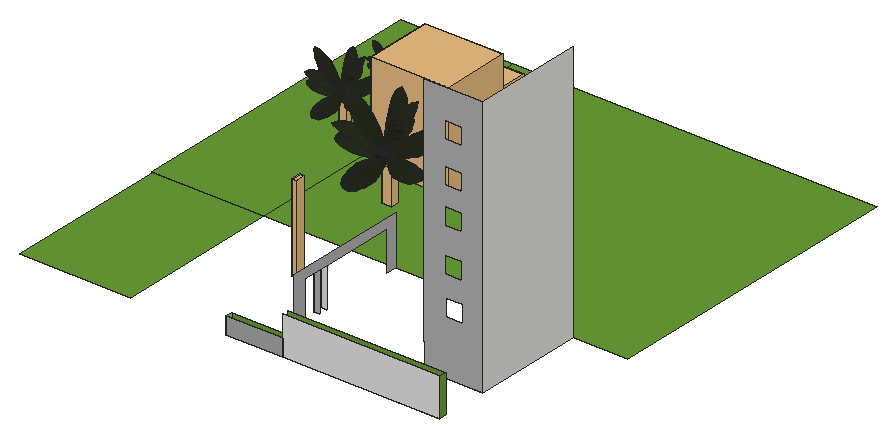
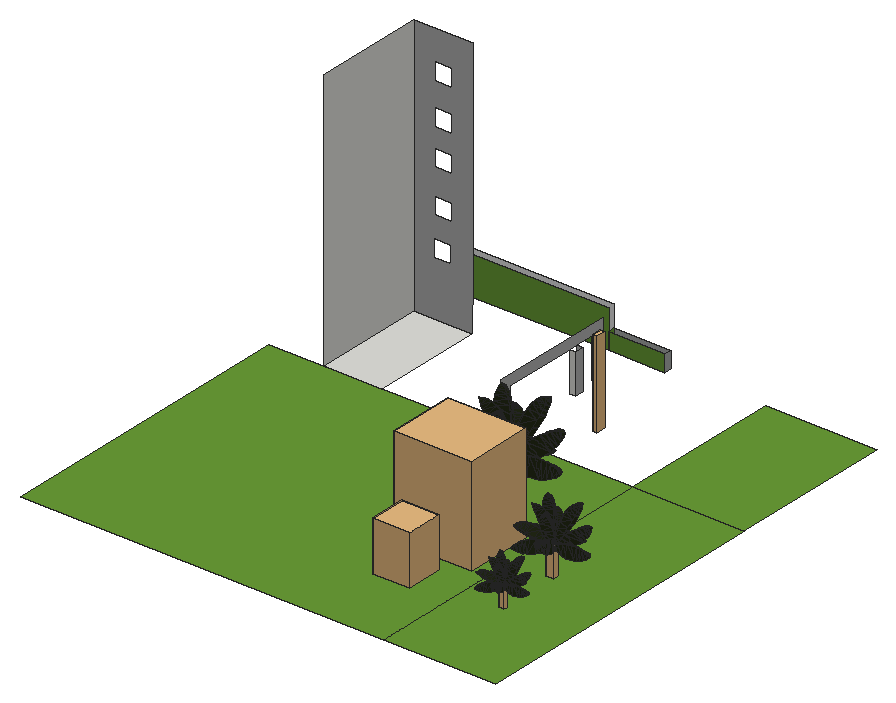
# SketchUp Ruby script. Lengths in inches.
U = 1.inch
M = Sketchup.active_model
def pt(a) = Geom::Point3d.new(a.map { |v| v * U })
def face(e, loops, mat)
  f = e.add_face(loops[0].map { |a| pt(a) })
  loops[1..].each { |l| e.add_face(l.map { |a| pt(a) }).erase! }
  f.material = f.back_material = mat if mat
  f
end
# faces: each face lists its corners as indices into pts; further lists are holes
def faces(e, pts, list, mat = nil) = list.each { |f| face(e, (f[0].is_a?(Array) ? f : [f]).map { |l| l.map { |i| pts[i] } }, mat) }
# xy, xz, yz: faces in a plane at the given z, y or x. An outline is a flat list of corners, or four numbers for a rectangle; further outlines are holes
def ring(l) = l.size == 4 ? [[l[0], l[1]], [l[2], l[1]], [l[2], l[3]], [l[0], l[3]]] : l.each_slice(2).to_a
def flat(e, list, mat, &to3) = list.each { |f| face(e, (f[0].is_a?(Array) ? f : [f]).map { |l| ring(l).map { |u, v| to3.(u, v) } }, mat) }
def xy(e, z, list, mat = nil) = flat(e, list, mat) { |x, y| [x, y, z] }
def xz(e, y, list, mat = nil) = flat(e, list, mat) { |x, z| [x, y, z] }
def yz(e, x, list, mat = nil) = flat(e, list, mat) { |y, z| [x, y, z] }
def lines(e, pts, list) = list.each { |a, b| e.add_line(pt(pts[a]), pt(pts[b])) }
# prism: a flat outline (further loops are holes) pulled along v
def prism(e, loops, v, mat = nil)
  f = face(e, loops, mat); d = Geom::Vector3d.new(v.map { |x| x * U })
  f.pushpull(f.normal.samedirection?(d) ? d.length : -d.length)
end
def box(e, o, s, mat = nil) = prism(e, [[o, [o[0] + s[0], o[1], o[2]], [o[0] + s[0], o[1] + s[1], o[2]], [o[0], o[1] + s[1], o[2]]]], [0, 0, s[2]], mat)
def at(x, y, z, deg = 0) = Geom::Transformation.translation(pt([x, y, z])) * Geom::Transformation.rotation(ORIGIN, Z_AXIS, deg.degrees)
def axes(o, x, y, z) = Geom::Transformation.new([*x, 0, *y, 0, *z, 0, *pt(o).to_a, 1])
def part(name) = M.definitions.add(name)
# library, detail: a bought-in or finely detailed component or shape, given as its bounding box
def library(name, o, s) = part(name).tap { |d| box(d.entities, o, s) }
def detail(e, o, s) = box(e.add_group.entities, o, s)
def put(e, d, t, mat = nil) = e.add_instance(d, t).tap { |i| i.material = mat if mat }
def group(e, t, mat = nil) = e.add_group.tap { |g| g.transformation = t; g.material = mat if mat }.entities
root = M.entities
M.materials.add("Niraj_Hair_Gray").color = [178, 178, 178]
M.materials.add("[Concrete Form 4x8]").color = [167, 170, 168]
M.materials.add("[Grass Dark Green]").color = [106, 157, 55]
M.materials.add("[Polished Concrete Old]").color = [229, 229, 229]
M.materials.add("cocoanut_mat").color = [137, 122, 109]
M.materials.add("cocoanut_scrub").color = [165, 152, 134]
M.materials.add("coconut_test3_clean").color = [38, 45, 24]
c1 = library("Small Tree",[-46.3125,-47.83,0],[89.1875,89.28,122.02])
c2 = part("coconut_half")
p = [[54.48,2.6,2.17],[90.24,0,0],[105.09,35.75,42.48],[115.87,5,0],[128.48,35.75,36.0625],[152.37,21,0],
  [152.37,35.75,27.13],[169.19,35.75,17.77],[57.93,35.75,46.59],[42.36,5.25,5.16],[79.93,35.75,46.59],[41.85,35.75,44.23],
  [28.04,8.5,7.49],[27.85,35.75,39.58],[16.59,14.5,9.63],[9.27,35.75,26.98],[6.26,23.5,11.78],[16.71,35.75,32.89],
  [0,35.75,14.25]]
faces(c2.entities,p,[[0,1,2],[1,3,4],[1,4,2],[3,5,6],[3,6,4],[5,7,6],[0,8,9],[0,10,8],
  [0,2,10],[9,11,12],[9,8,11],[12,13,14],[12,11,13],[14,15,16],[14,17,15],[14,13,17],
  [18,16,15]],"coconut_test3_clean")
c3 = part("Group\#8")
put(c3.entities,c2,at(0,0,0))
put(c3.entities,c2,axes([0,71.5,0],[1,0,0],[0,-1,0],[0,0,1]))
c4 = part("coconut3_top")
put(c4.entities,c3,axes([-176.42,-40.5625,245.57],[1,0,0],[0,0.96593,-0.25882],[0,0.25882,0.96593]))
g1 = group(c4.entities,at(-4.7,-151.6,178.32))
put(g1,c2,axes([0,0,0],[0.14944,0.9543,0.25882],[-0.87562,0.00613,0.48296],[0.4593,-0.2988,0.83652]))
put(g1,c2,axes([-62.61,0.4375,34.53],[0.14944,0.9543,0.25882],[0.87562,-0.00613,-0.48296],[0.4593,-0.2988,0.83652]))
put(c4.entities,c3,axes([171.02,-15.64,245.06],[-0.94665,0.32227,0],[-0.31128,-0.91439,-0.25882],[-0.08341,-0.24501,0.96593]))
put(c4.entities,c3,axes([41.29,183.8,264.73],[-0.39574,-0.90582,-0.15126],[0.91636,-0.40035,0],[-0.06056,-0.13861,0.98849]))
put(c4.entities,c3,axes([-77.19,156.92,280.49],[0.30009,-0.91813,-0.25882],[0.86338,0.14605,0.48296],[-0.40562,-0.36839,0.83652]))
put(c4.entities,c3,axes([-112.56,-104.35,340.4],[0.76036,0.41456,-0.5],[-0.63406,0.64068,-0.43301],[0.14083,0.64627,0.75]))
put(c4.entities,c3,axes([119.49,-113.07,311.83],[-0.54618,0.67208,-0.5],[-0.83762,-0.43208,0.3342],[0.00857,0.60135,0.79894]))
put(c4.entities,c3,axes([103.27,116.54,337.13],[-0.75167,-0.49748,-0.43301],[0.65951,-0.56129,-0.5],[0.0057,-0.66141,0.75]))
put(c4.entities,c3,axes([-111.91,-75.47,434.48],[0.55528,0.30275,-1.09544],[-0.10884,0.68367,0.13377],[0.95166,0.05419,0.49738]))
put(c4.entities,c3,axes([96.22,-37.8,421.8],[-0.43628,0.34579,-0.96422],[-0.35338,-0.74638,-0.10777],[-0.75439,0.29273,0.44631]))
put(c4.entities,c3,axes([-41.59,80.66,420.02],[0.06101,-0.43197,-0.99256],[0.722,0.18761,-0.03727],[0.23024,-0.81295,0.36796]))
put(c4.entities,c3,axes([62.57,69.42,421.8],[-0.49424,-0.25619,-0.96422],[0.53593,-0.62829,-0.10777],[-0.57624,-0.5681,0.44631]))
c5 = part("cocoanut_mat")
yz(c5.entities,2,[[0.45,5,4.17,5,4.55,7.22,0,7.22]],"cocoanut_mat")
p = [[1.5,0.95,2.55],[0,1.26,0],[1.5,4.17,2.55],[0,3.01,0.06],[2,0.45,5],[2,4.17,5],
  [1.5,4.82,10.82],[1.5,0,9.97],[2,4.55,7.22],[2,0,7.22],[1,0.99,11.1],[1,3.98,11.36]]
faces(c5.entities,p,[[0,1,2],[3,2,1],[4,0,2,5],[6,7,8],[9,8,7],[7,6,10],[11,10,6]],"cocoanut_mat")
c6 = part("Coconut Palm")
xy(c6.entities,112.14,[[122.28,106.09,125.08,107.25,126.24,110.05,125.08,112.85,122.28,114.01,119.48,112.85,118.32,110.05,119.48,107.25]])
detail(c6.entities,[118.32,101.24,0],[25.61,17.45,83.17])
put(c6.entities,c4,axes([125.26,110.5,-76.06],[0.71,0,0],[0,0.71,0],[0,0,0.71]))
g2 = group(c6.entities,at(117.6,103.69,82.125))
p = [[4.68,2.4,1.05],[4.68,2.4,30.02],[1.88,3.56,30.02],[1.88,3.56,1.05],[7.48,3.56,1.05],[7.48,3.56,30.02],
  [0.72,6.36,30.02],[0.72,6.36,1.05],[8.64,6.36,1.05],[8.64,6.36,30.02],[1.88,9.16,30.02],[1.88,9.16,1.05],
  [7.48,9.16,1.05],[7.48,9.16,30.02],[4.68,10.32,30.02],[4.68,10.32,1.05]]
faces(g2,p,[[0,1,2,3],[4,5,1,0],[2,6,7,3],[4,8,9,5],[6,10,11,7],[8,12,13,9],[11,10,14,15],[15,14,13,12]],"cocoanut_scrub")
put(g2,c5,axes([8.73,9,14.81],[0.95137,0.17914,0.2506],[-0.24236,0.93742,0.25],[-0.19013,-0.29858,0.93525]))
put(g2,c5,axes([1.89,13.92,14.26],[-0.95388,0.23795,0.18301],[-0.27087,-0.94506,-0.18301],[0.17341,-0.30035,1.29434]))
put(g2,c5,axes([3.98,0.08,4.09],[0.521,-0.82169,0.23104],[0.85353,0.50368,-0.13339],[-0.00676,0.2667,0.96376]))
put(g2,c5,axes([2.8,2.4,6.76],[-0.16755,-0.98247,0.08171],[0.984,-0.16156,0.07513],[-0.09879,0.15157,1.61993]))
put(g2,c5,axes([8.29,10.47,4.97],[0.02489,0.99575,0.08868],[-0.99708,0.03112,-0.06968],[-0.11254,-0.13523,1.55005]))
put(g2,c5,axes([10.54,2.88,6.76],[0.95137,0.17914,0.2506],[-0.115,0.96125,-0.25056],[-0.28577,0.20956,0.9351]))
c7 = library("trunk\#1",[0,0,0],[11.46,27.17,238.43])
c8 = library("Group\#102",[-22.47,-14.25,0],[191.27,167.9,240.05])
xy(root,0,[[645.65,57.05,1032.97,75.24],[890.84,187.625,1032.97,464.11]])
xy(root,0,[[2.96,57.05,275.09,464.11],[0,464.11,275.09,1226.8],[275.09,464.11,1166.9,1226.8]],"[Grass Dark Green]")
xz(root,57.05,[[506.24,0,645.65,40.75]],"[Concrete Form 4x8]")
xz(root,57.05,[[645.65,0,1032.97,93.8125]],"[Polished Concrete Old]")
xz(root,75.24,[[506.24,0,645.65,40.75],[645.65,0,1032.97,93.8125]],"[Grass Dark Green]")
xz(root,187.625,[[[890.84,0,1032.97,0,1032.97,639.04,888.71,639.04,888.71,124.25],[939.31,228.57,981.74,271],[939.31,334.38,981.74,376.82],[939.31,422.88,981.74,465.32],[939.31,523.94,981.74,566.38],[941.43,134.5,983.87,176.94]]],"Niraj_Hair_Gray")
xz(root,233.07,[[582.23,0,597.61,97.1875]],"Niraj_Hair_Gray")
xz(root,254.44,[[582.23,0,597.61,97.3125]])
yz(root,506.24,[[57.05,0,75.24,40.75]],"[Concrete Form 4x8]")
yz(root,582.23,[[233.07,0,254.44,97.3125]],"Niraj_Hair_Gray")
yz(root,597.61,[[153,0,153,121.74,464.11,121.74,464.11,0,437.85,0,437.85,97.125,254.44,97.125,254.44,97.3125,233.07,97.3125,233.07,97.1875,186.88,97.1875,186.88,0]],"Niraj_Hair_Gray")
yz(root,645.65,[[57.05,0,75.24,40.75]],"[Grass Dark Green]")
yz(root,1032.97,[[187.625,0,464.11,639.04]])
yz(root,1032.97,[[57.05,0,75.24,93.8125]],"[Grass Dark Green]")
put(root,c1,at(409.57,997.1,0))
put(root,c6,axes([88.13,754.08,0],[0.7,0,0],[0,0.7,0],[0,0,0.7]))
put(root,c6,axes([113.24,932.72,0],[0.483,0,0],[0,0.483,0],[0,0,0.483]))
put(root,c7,axes([461.99,317.1,0],[0.89,0,0],[0,0.89,0],[0,0,0.89]))
put(root,c8,at(334.47,758.88,0))
put(root,c6,at(299.12,545.36,0))
